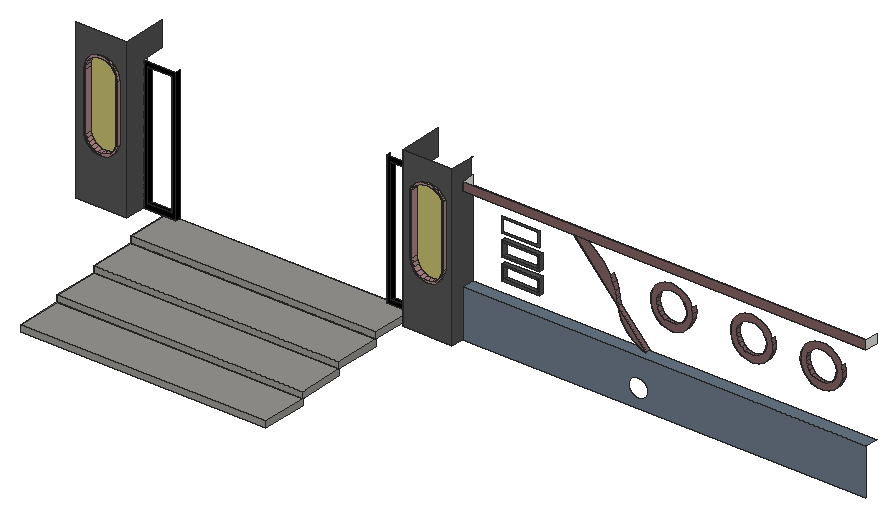
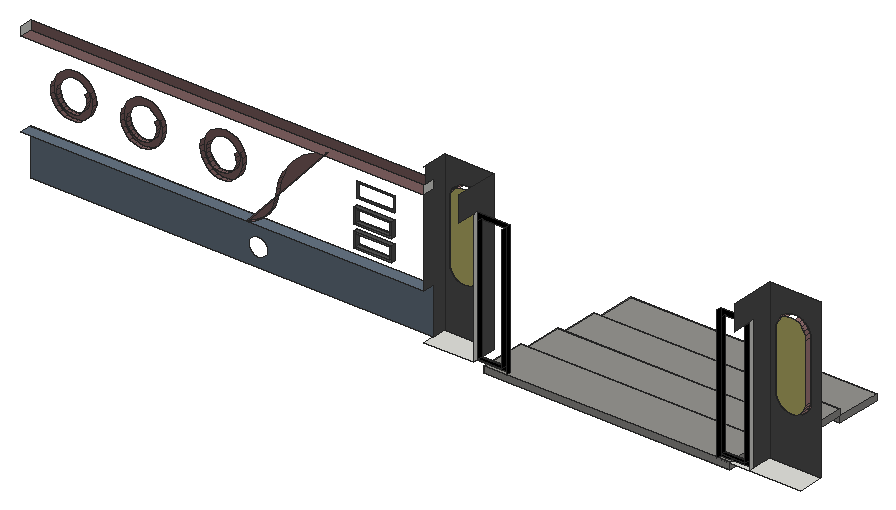
# SketchUp Ruby script. Lengths in inches.
U = 1.inch
M = Sketchup.active_model
def pt(a) = Geom::Point3d.new(a.map { |v| v * U })
def face(e, loops, mat)
  f = e.add_face(loops[0].map { |a| pt(a) })
  loops[1..].each { |l| e.add_face(l.map { |a| pt(a) }).erase! }
  f.material = f.back_material = mat if mat
  f
end
# faces: each face lists its corners as indices into pts; further lists are holes
def faces(e, pts, list, mat = nil) = list.each { |f| face(e, (f[0].is_a?(Array) ? f : [f]).map { |l| l.map { |i| pts[i] } }, mat) }
# xy, xz, yz: faces in a plane at the given z, y or x. An outline is a flat list of corners, or four numbers for a rectangle; further outlines are holes
def ring(l) = l.size == 4 ? [[l[0], l[1]], [l[2], l[1]], [l[2], l[3]], [l[0], l[3]]] : l.each_slice(2).to_a
def flat(e, list, mat, &to3) = list.each { |f| face(e, (f[0].is_a?(Array) ? f : [f]).map { |l| ring(l).map { |u, v| to3.(u, v) } }, mat) }
def xy(e, z, list, mat = nil) = flat(e, list, mat) { |x, y| [x, y, z] }
def xz(e, y, list, mat = nil) = flat(e, list, mat) { |x, z| [x, y, z] }
def yz(e, x, list, mat = nil) = flat(e, list, mat) { |y, z| [x, y, z] }
def lines(e, pts, list) = list.each { |a, b| e.add_line(pt(pts[a]), pt(pts[b])) }
# prism: a flat outline (further loops are holes) pulled along v
def prism(e, loops, v, mat = nil)
  f = face(e, loops, mat); d = Geom::Vector3d.new(v.map { |x| x * U })
  f.pushpull(f.normal.samedirection?(d) ? d.length : -d.length)
end
def box(e, o, s, mat = nil) = prism(e, [[o, [o[0] + s[0], o[1], o[2]], [o[0] + s[0], o[1] + s[1], o[2]], [o[0], o[1] + s[1], o[2]]]], [0, 0, s[2]], mat)
def at(x, y, z, deg = 0) = Geom::Transformation.translation(pt([x, y, z])) * Geom::Transformation.rotation(ORIGIN, Z_AXIS, deg.degrees)
def axes(o, x, y, z) = Geom::Transformation.new([*x, 0, *y, 0, *z, 0, *pt(o).to_a, 1])
def part(name) = M.definitions.add(name)
# library, detail: a bought-in or finely detailed component or shape, given as its bounding box
def library(name, o, s) = part(name).tap { |d| box(d.entities, o, s) }
def detail(e, o, s) = box(e.add_group.entities, o, s)
def put(e, d, t, mat = nil) = e.add_instance(d, t).tap { |i| i.material = mat if mat }
def group(e, t, mat = nil) = e.add_group.tap { |g| g.transformation = t; g.material = mat if mat }.entities
root = M.entities
M.materials.add("[0057_DarkKhaki]1").color = [189, 183, 107]
M.materials.add("[0111_SlateGray]").color = [103, 117, 132]
M.materials.add("[0119_RosyBrown]1").color = [124, 95, 95]
M.materials.add("[0119_RosyBrown]2").color = [170, 129, 129]
M.materials.add("[0135_DarkGray]").color = [81, 81, 81]
M.materials.add("[0137_Black]").color = [0, 0, 0]
M.materials.add("[Granite Light Gray]").color = [149, 148, 144]
xy(root,0,[[7,639.11,31.33,651.11],[162.58,639.11,186.0625,651.11],[31.33,649.11,46.92,651.11]])
xy(root,2.07,[[149.02,649.11,160.48,651.11]],"[0137_Black]")
xy(root,2.3,[[33.63,649.11,44.62,651.11]],"[0137_Black]")
xy(root,22.19,[[186.0625,645.11,377.9375,651.11]],"[0111_SlateGray]")
xy(root,28.6875,[[201.56,649.11,219.5,651.11]],"[0135_DarkGray]")
xy(root,29.54,[[202.42,649.11,218.64,651.11]],"[0135_DarkGray]")
xy(root,35.08,[[202.42,649.11,218.64,651.11]],"[0135_DarkGray]")
xy(root,35.9375,[[201.56,649.11,219.5,651.11]],"[0135_DarkGray]")
xy(root,38.875,[[201.56,649.11,219.5,651.11]],"[0135_DarkGray]")
xy(root,39.62,[[202.31,649.11,218.75,651.11]],"[0135_DarkGray]")
xy(root,45.375,[[202.31,649.11,218.75,651.11]],"[0135_DarkGray]")
xy(root,46.125,[[201.56,649.11,219.5,651.11]],"[0135_DarkGray]")
xy(root,63,[[186.0625,645.11,377.9375,651.11]],"[0119_RosyBrown]1")
xz(root,638.11,[[[19.87,22.97,21.71,23.18,23.47,23.8,25.04,24.79,26.34,26.11,27.32,27.6875,27.94,29.49,27.94,57.27,27.67,59.36,26.86,61.31,25.58,62.98,23.9,64.26,21.96,65.07,19.87,65.35,17.78,65.07,15.83,64.26,14.16,62.98,12.875,61.31,12.07,59.36,11.79,57.27,11.79,29.49,12.41,27.6875,13.39,26.11,14.7,24.79,16.27,23.8,18.02,23.18],[19.87,23.86,18.22,24.05,16.66,24.6,15.26,25.49,14.09,26.66,13.22,28.07,12.68,29.64,12.68,57.27,12.92,59.13,13.64,60.87,14.79,62.35,16.27,63.5,18.01,64.21,19.87,64.46,21.73,64.21,23.46,63.5,24.95,62.35,26.09,60.87,26.81,59.13,27.05,57.27,27.05,29.64,26.52,28.07,25.64,26.66,24.48,25.49,23.08,24.6,21.51,24.05]],[[174.87,23.28,176.93,23.55,178.86,24.35,180.51,25.62,181.78,27.27,182.58,29.19,182.85,31.26,182.85,60.6,181.89,62.1,180.79,63.28,179.49,64.24,178.04,64.95,176.48,65.39,174.87,65.54,173.26,65.39,171.7,64.95,170.25,64.24,168.95,63.28,167.84,62.1,166.88,60.6,166.88,31.26,167.16,29.19,167.95,27.27,169.22,25.62,170.875,24.35,172.8,23.55],[174.87,24.07,173.01,24.32,171.27,25.04,169.79,26.18,168.64,27.67,167.92,29.4,167.68,31.26,167.68,60.37,168.47,61.61,169.48,62.68,170.66,63.56,171.98,64.21,173.4,64.6,174.87,64.74,176.33,64.6,177.75,64.21,179.07,63.56,180.26,62.68,181.26,61.61,182.05,60.37,182.05,31.26,181.81,29.4,181.09,27.67,179.95,26.18,178.46,25.04,176.73,24.32]]],"[0119_RosyBrown]2")
xz(root,639.11,[[[7,0,31.33,75],[19.87,22.97,18.02,23.18,16.27,23.8,14.7,24.79,13.39,26.11,12.41,27.6875,11.79,29.49,11.79,57.27,12.07,59.36,12.875,61.31,14.16,62.98,15.83,64.26,17.78,65.07,19.87,65.35,21.96,65.07,23.9,64.26,25.58,62.98,26.86,61.31,27.67,59.36,27.94,57.27,27.94,29.49,27.32,27.6875,26.34,26.11,25.04,24.79,23.47,23.8,21.71,23.18]],[[162.58,0,186.0625,75],[174.87,23.28,172.8,23.55,170.875,24.35,169.22,25.62,167.95,27.27,167.16,29.19,166.88,31.26,166.88,60.6,167.84,62.1,168.95,63.28,170.25,64.24,171.7,64.95,173.26,65.39,174.87,65.54,176.48,65.39,178.04,64.95,179.49,64.24,180.79,63.28,181.89,62.1,182.85,60.6,182.85,31.26,182.58,29.19,181.78,27.27,180.51,25.62,178.86,24.35,176.93,23.55]]],"[0135_DarkGray]")
xz(root,641.11,[[19.87,23.86,21.51,24.05,23.08,24.6,24.48,25.49,25.64,26.66,26.52,28.07,27.05,29.64,27.05,57.27,26.81,59.13,26.09,60.87,24.95,62.35,23.46,63.5,21.73,64.21,19.87,64.46,18.01,64.21,16.27,63.5,14.79,62.35,13.64,60.87,12.92,59.13,12.68,57.27,12.68,29.64,13.22,28.07,14.09,26.66,15.26,25.49,16.66,24.6,18.22,24.05],[174.87,24.07,176.73,24.32,178.46,25.04,179.95,26.18,181.09,27.67,181.81,29.4,182.05,31.26,182.05,60.37,181.26,61.61,180.26,62.68,179.07,63.56,177.75,64.21,176.33,64.6,174.87,64.74,173.4,64.6,171.98,64.21,170.66,63.56,169.48,62.68,168.47,61.61,167.68,60.37,167.68,31.26,167.92,29.4,168.64,27.67,169.79,26.18,171.27,25.04,173.01,24.32]],"[0057_DarkKhaki]1")
xz(root,645.11,[[[186.0625,0,377.9375,22.19],[269.68,4.18,268.52,4.33,267.43,4.78,266.5,5.5,265.79,6.43,265.34,7.52,265.18,8.68,265.34,9.85,265.79,10.93,266.5,11.86,267.43,12.58,268.52,13.03,269.68,13.18,270.85,13.03,271.93,12.58,272.87,11.86,273.58,10.93,274.03,9.85,274.18,8.68,274.03,7.52,273.58,6.43,272.87,5.5,271.93,4.78,270.85,4.33]]],"[0111_SlateGray]")
xz(root,645.11,[[186.0625,63,377.9375,67.2]],"[0119_RosyBrown]1")
xz(root,649.11,[[270.01,22.19,270.11,22.28,256.72,37.33,256.61,37.24,256.97,35.5,257.5,33.8125,258.1875,32.18,259.02,30.61,260,29.14,261.12,27.76,262.36,26.49,263.71,25.35,265.17,24.34,266.71,23.47,268.33,22.75],[[282.96,35.68,285.56,36.18,287.93,37.34,289.93,39.07,291.41,41.26,292.27,43.76,292.46,46.4,291.95,48.99,290.8,51.37,289.0625,53.37,286.875,54.85,284.375,55.71,281.74,55.9,279.14,55.39,276.77,54.24,274.77,52.5,273.29,50.3125,272.43,47.8125,272.24,45.18,272.75,42.58,273.9,40.21,275.64,38.21,277.83,36.73,280.32,35.87],[282.78,38.68,280.92,38.81,279.17,39.41,277.625,40.46,276.41,41.86,275.59,43.53,275.24,45.36,275.37,47.21,275.98,48.97,277.02,50.51,278.42,51.73,280.09,52.55,281.92,52.9,283.77,52.77,285.53,52.16,287.07,51.12,288.29,49.72,289.11,48.04,289.46,46.22,289.33,44.36,288.72,42.6,287.68,41.0625,286.28,39.84,284.61,39.03]],[[320.9,35.68,323.49,36.18,325.87,37.34,327.87,39.07,329.35,41.26,330.21,43.76,330.39,46.4,329.89,48.99,328.73,51.37,327,53.37,324.8125,54.85,322.3125,55.71,319.68,55.9,317.08,55.39,314.7,54.24,312.71,52.5,311.23,50.3125,310.37,47.8125,310.18,45.18,310.68,42.58,311.84,40.21,313.57,38.21,315.76,36.73,318.26,35.87],[320.72,38.68,318.86,38.81,317.1,39.41,315.5625,40.46,314.34,41.86,313.53,43.53,313.18,45.36,313.31,47.21,313.91,48.97,314.95,50.51,316.36,51.73,318.03,52.55,319.86,52.9,321.71,52.77,323.47,52.16,325.01,51.12,326.23,49.72,327.05,48.04,327.4,46.22,327.27,44.36,326.66,42.6,325.62,41.0625,324.22,39.84,322.54,39.03]],[[354.15,35.68,356.74,36.18,359.12,37.34,361.12,39.07,362.6,41.26,363.46,43.76,363.64,46.4,363.14,48.99,361.98,51.37,360.25,53.37,358.0625,54.85,355.5625,55.71,352.93,55.9,350.33,55.39,347.95,54.24,345.96,52.5,344.48,50.3125,343.62,47.8125,343.43,45.18,343.93,42.58,345.09,40.21,346.82,38.21,349.01,36.73,351.51,35.87],[353.97,38.68,352.11,38.81,350.35,39.41,348.8125,40.46,347.59,41.86,346.78,43.53,346.43,45.36,346.56,47.21,347.16,48.97,348.2,50.51,349.61,51.73,351.28,52.55,353.11,52.9,354.96,52.77,356.72,52.16,358.26,51.12,359.48,49.72,360.3,48.04,360.65,46.22,360.52,44.36,359.91,42.6,358.87,41.0625,357.47,39.84,355.79,39.03]],[256.61,37.24,256.26,40.32,255.56,43.34,254.54,46.26,253.19,49.06,251.55,51.68,249.62,54.11,247.43,56.31,245.01,58.24,242.39,59.9,239.6,61.26,236.68,62.29,233.66,63]],"[0119_RosyBrown]1")
xz(root,649.11,[[[201.56,28.6875,219.5,35.9375],[202.42,29.54,218.64,35.08]],[[201.56,38.875,219.5,46.125],[202.31,39.62,218.75,45.375]],[[201.56,49.0625,219.5,56.3125],[202.32,49.82,218.74,55.55]]],"[0135_DarkGray]")
xz(root,649.11,[[[31.33,0,46.92,63],[33.63,2.3,44.62,60.7]],[[146.95,0,162.54,63],[149.02,2.07,160.48,60.93]]],"[0137_Black]")
yz(root,11.79,[[638.11,29.49,639.11,57.27]])
yz(root,12.68,[[638.11,29.64,641.11,57.27]],"[0119_RosyBrown]2")
yz(root,27.05,[[638.11,29.64,641.11,57.27]],"[0119_RosyBrown]2")
yz(root,27.94,[[638.11,29.49,639.11,57.27]],"[0119_RosyBrown]2")
yz(root,31.33,[[649.11,0,651.11,63]])
yz(root,31.33,[[639.11,0,649.11,0,649.11,63,660.11,63,660.11,75,639.11,75]],"[0135_DarkGray]")
yz(root,33.63,[[649.11,2.3,651.11,60.7]],"[0137_Black]")
yz(root,44.62,[[649.11,2.3,651.11,60.7]],"[0137_Black]")
yz(root,46.92,[[649.11,0,651.11,63]],"[0137_Black]")
yz(root,146.95,[[649.11,0,651.11,63]],"[0137_Black]")
yz(root,149.02,[[649.11,2.07,651.11,60.93]],"[0137_Black]")
yz(root,160.48,[[649.11,2.07,651.11,60.93]],"[0137_Black]")
yz(root,162.54,[[649.11,0,651.11,63]])
yz(root,162.58,[[639.11,0,639.11,75,660.11,75,660.11,63,651.11,63,651.11,0]],"[0135_DarkGray]")
yz(root,166.88,[[638.11,31.26,639.11,60.6]],"[0119_RosyBrown]2")
yz(root,167.68,[[638.11,31.26,641.11,60.37]],"[0119_RosyBrown]2")
yz(root,182.05,[[638.11,31.26,641.11,60.37]],"[0119_RosyBrown]2")
yz(root,182.85,[[638.11,31.26,639.11,60.6]],"[0119_RosyBrown]2")
yz(root,186.0625,[[645.11,63,651.11,67.2]])
yz(root,186.0625,[[639.11,0,645.11,0,645.11,22.19,651.11,22.19,651.11,63,645.11,63,645.11,67.2,650.11,67.2,650.11,74.96,651.11,74.96,651.11,75,639.11,75]],"[0135_DarkGray]")
yz(root,201.56,[[649.11,28.6875,651.11,35.9375],[649.11,38.875,651.11,46.125]],"[0135_DarkGray]")
yz(root,202.31,[[649.11,39.62,651.11,45.375]],"[0135_DarkGray]")
yz(root,202.42,[[649.11,29.54,651.11,35.08]],"[0135_DarkGray]")
yz(root,218.64,[[649.11,29.54,651.11,35.08]],"[0135_DarkGray]")
yz(root,218.75,[[649.11,39.62,651.11,45.375]],"[0135_DarkGray]")
yz(root,219.5,[[649.11,28.6875,651.11,35.9375],[649.11,38.875,651.11,46.125]],"[0135_DarkGray]")
yz(root,377.9375,[[645.11,63,651.11,67.2]])
p = [[268.33,651.11,22.75],[270.01,651.11,22.19],[270.01,649.11,22.19],[268.33,649.11,22.75],[270.11,651.11,22.28],[270.11,649.11,22.28],
  [256.72,651.11,37.33],[256.72,649.11,37.33],[266.71,651.11,23.47],[266.71,649.11,23.47],[18.02,639.11,23.18],[19.87,639.11,22.97],
  [19.87,638.11,22.97],[18.02,638.11,23.18],[21.71,639.11,23.18],[21.71,638.11,23.18],[16.27,639.11,23.8],[16.27,638.11,23.8],
  [23.47,639.11,23.8],[23.47,638.11,23.8],[172.8,639.11,23.55],[174.87,639.11,23.28],[174.87,638.11,23.28],[172.8,638.11,23.55],
  [176.93,639.11,23.55],[176.93,638.11,23.55],[170.875,639.11,24.35],[170.875,638.11,24.35],[178.86,639.11,24.35],[178.86,638.11,24.35],
  [265.17,651.11,24.34],[265.17,649.11,24.34],[14.7,639.11,24.79],[14.7,638.11,24.79],[25.04,639.11,24.79],[25.04,638.11,24.79],
  [18.22,641.11,24.05],[18.22,638.11,24.05],[19.87,638.11,23.86],[19.87,641.11,23.86],[21.51,638.11,24.05],[21.51,641.11,24.05],
  [16.66,641.11,24.6],[16.66,638.11,24.6],[23.08,638.11,24.6],[23.08,641.11,24.6],[173.01,641.11,24.32],[173.01,638.11,24.32],
  [174.87,638.11,24.07],[174.87,641.11,24.07],[176.73,638.11,24.32],[176.73,641.11,24.32],[169.22,639.11,25.62],[169.22,638.11,25.62],
  [171.27,641.11,25.04],[171.27,638.11,25.04],[178.46,638.11,25.04],[178.46,641.11,25.04],[180.51,639.11,25.62],[180.51,638.11,25.62],
  [263.71,651.11,25.35],[263.71,649.11,25.35],[15.26,641.11,25.49],[15.26,638.11,25.49],[24.48,638.11,25.49],[24.48,641.11,25.49],
  [13.39,639.11,26.11],[13.39,638.11,26.11],[26.34,639.11,26.11],[26.34,638.11,26.11],[169.79,641.11,26.18],[169.79,638.11,26.18],
  [179.95,638.11,26.18],[179.95,641.11,26.18],[262.36,651.11,26.49],[262.36,649.11,26.49],[14.09,641.11,26.66],[14.09,638.11,26.66],
  [25.64,638.11,26.66],[25.64,641.11,26.66],[167.95,639.11,27.27],[167.95,638.11,27.27],[181.78,639.11,27.27],[181.78,638.11,27.27],
  [12.41,639.11,27.6875],[12.41,638.11,27.6875],[27.32,639.11,27.6875],[27.32,638.11,27.6875],[168.64,641.11,27.67],[168.64,638.11,27.67],
  [181.09,638.11,27.67],[181.09,641.11,27.67],[261.12,651.11,27.76],[261.12,649.11,27.76],[13.22,641.11,28.07],[13.22,638.11,28.07],
  [26.52,638.11,28.07],[26.52,641.11,28.07],[167.16,639.11,29.19],[167.16,638.11,29.19],[182.58,639.11,29.19],[182.58,638.11,29.19],
  [11.79,639.11,29.49],[11.79,638.11,29.49],[27.94,639.11,29.49],[27.94,638.11,29.49],[167.92,641.11,29.4],[167.92,638.11,29.4],
  [181.81,638.11,29.4],[181.81,641.11,29.4],[260,651.11,29.14],[260,649.11,29.14],[12.68,641.11,29.64],[12.68,638.11,29.64],
  [27.05,638.11,29.64],[27.05,641.11,29.64],[259.02,651.11,30.61],[259.02,649.11,30.61],[166.88,639.11,31.26],[166.88,638.11,31.26],
  [182.85,639.11,31.26],[182.85,638.11,31.26],[167.68,641.11,31.26],[167.68,638.11,31.26],[182.05,638.11,31.26],[182.05,641.11,31.26],
  [258.1875,651.11,32.18],[258.1875,649.11,32.18],[257.5,651.11,33.8125],[257.5,649.11,33.8125],[256.97,651.11,35.5],[256.97,649.11,35.5],
  [256.61,651.11,37.24],[256.61,649.11,37.24],[280.32,651.11,35.87],[282.96,651.11,35.68],[282.96,649.11,35.68],[280.32,649.11,35.87],
  [285.56,651.11,36.18],[285.56,649.11,36.18],[318.26,651.11,35.87],[320.9,651.11,35.68],[320.9,649.11,35.68],[318.26,649.11,35.87],
  [323.49,651.11,36.18],[323.49,649.11,36.18],[351.51,651.11,35.87],[354.15,651.11,35.68],[354.15,649.11,35.68],[351.51,649.11,35.87],
  [356.74,651.11,36.18],[356.74,649.11,36.18],[277.83,651.11,36.73],[277.83,649.11,36.73],[315.76,651.11,36.73],[315.76,649.11,36.73],
  [349.01,651.11,36.73],[349.01,649.11,36.73],[287.93,651.11,37.34],[287.93,649.11,37.34],[325.87,651.11,37.34],[325.87,649.11,37.34],
  [359.12,651.11,37.34],[359.12,649.11,37.34],[275.64,651.11,38.21],[275.64,649.11,38.21],[313.57,651.11,38.21],[313.57,649.11,38.21],
  [346.82,651.11,38.21],[346.82,649.11,38.21],[233.66,651.11,63],[233.66,649.11,63],[256.26,651.11,40.32],[256.26,649.11,40.32],
  [289.93,651.11,39.07],[289.93,649.11,39.07],[327.87,651.11,39.07],[327.87,649.11,39.07],[361.12,651.11,39.07],[361.12,649.11,39.07],
  [273.9,651.11,40.21],[273.9,649.11,40.21],[311.84,651.11,40.21],[311.84,649.11,40.21],[345.09,651.11,40.21],[345.09,649.11,40.21],
  [282.78,651.11,38.68],[280.92,651.11,38.81],[280.92,649.11,38.81],[282.78,649.11,38.68],[284.61,651.11,39.03],[284.61,649.11,39.03],
  [320.72,651.11,38.68],[318.86,651.11,38.81],[318.86,649.11,38.81],[320.72,649.11,38.68],[322.54,651.11,39.03],[322.54,649.11,39.03],
  [353.97,651.11,38.68],[352.11,651.11,38.81],[352.11,649.11,38.81],[353.97,649.11,38.68],[355.79,651.11,39.03],[355.79,649.11,39.03],
  [279.17,651.11,39.41],[279.17,649.11,39.41],[317.1,651.11,39.41],[317.1,649.11,39.41],[350.35,651.11,39.41],[350.35,649.11,39.41],
  [286.28,651.11,39.84],[286.28,649.11,39.84],[324.22,651.11,39.84],[324.22,649.11,39.84],[357.47,651.11,39.84],[357.47,649.11,39.84],
  [291.41,651.11,41.26],[291.41,649.11,41.26],[329.35,651.11,41.26],[329.35,649.11,41.26],[362.6,651.11,41.26],[362.6,649.11,41.26],
  [277.625,651.11,40.46],[277.625,649.11,40.46],[315.5625,651.11,40.46],[315.5625,649.11,40.46],[348.8125,651.11,40.46],[348.8125,649.11,40.46],
  [287.68,651.11,41.0625],[287.68,649.11,41.0625],[325.62,651.11,41.0625],[325.62,649.11,41.0625],[358.87,651.11,41.0625],[358.87,649.11,41.0625],
  [272.75,651.11,42.58],[272.75,649.11,42.58],[310.68,651.11,42.58],[310.68,649.11,42.58],[343.93,651.11,42.58],[343.93,649.11,42.58],
  [255.56,651.11,43.34],[255.56,649.11,43.34],[276.41,651.11,41.86],[276.41,649.11,41.86],[314.34,651.11,41.86],[314.34,649.11,41.86],
  [347.59,651.11,41.86],[347.59,649.11,41.86],[288.72,651.11,42.6],[288.72,649.11,42.6],[326.66,651.11,42.6],[326.66,649.11,42.6],
  [359.91,651.11,42.6],[359.91,649.11,42.6],[292.27,651.11,43.76],[292.27,649.11,43.76],[330.21,651.11,43.76],[330.21,649.11,43.76],
  [363.46,651.11,43.76],[363.46,649.11,43.76],[275.59,651.11,43.53],[275.59,649.11,43.53],[313.53,651.11,43.53],[313.53,649.11,43.53],
  [346.78,651.11,43.53],[346.78,649.11,43.53],[272.24,651.11,45.18],[272.24,649.11,45.18],[289.33,651.11,44.36],[289.33,649.11,44.36],
  [310.18,651.11,45.18],[310.18,649.11,45.18],[327.27,651.11,44.36],[327.27,649.11,44.36],[343.43,651.11,45.18],[343.43,649.11,45.18],
  [360.52,651.11,44.36],[360.52,649.11,44.36],[254.54,651.11,46.26],[254.54,649.11,46.26],[275.24,651.11,45.36],[275.24,649.11,45.36],
  [313.18,651.11,45.36],[313.18,649.11,45.36],[346.43,651.11,45.36],[346.43,649.11,45.36],[292.46,651.11,46.4],[292.46,649.11,46.4],
  [330.39,651.11,46.4],[330.39,649.11,46.4],[363.64,651.11,46.4],[363.64,649.11,46.4],[289.46,651.11,46.22],[289.46,649.11,46.22],
  [327.4,651.11,46.22],[327.4,649.11,46.22],[360.65,651.11,46.22],[360.65,649.11,46.22],[272.43,651.11,47.8125],[272.43,649.11,47.8125],
  [310.37,651.11,47.8125],[310.37,649.11,47.8125],[343.62,651.11,47.8125],[343.62,649.11,47.8125],[275.37,651.11,47.21],[275.37,649.11,47.21],
  [313.31,651.11,47.21],[313.31,649.11,47.21],[346.56,651.11,47.21],[346.56,649.11,47.21],[289.11,651.11,48.04],[289.11,649.11,48.04],
  [327.05,651.11,48.04],[327.05,649.11,48.04],[360.3,651.11,48.04],[360.3,649.11,48.04],[253.19,651.11,49.06],[253.19,649.11,49.06],
  [291.95,651.11,48.99],[291.95,649.11,48.99],[329.89,651.11,48.99],[329.89,649.11,48.99],[363.14,651.11,48.99],[363.14,649.11,48.99],
  [275.98,651.11,48.97],[275.98,649.11,48.97],[313.91,651.11,48.97],[313.91,649.11,48.97],[347.16,651.11,48.97],[347.16,649.11,48.97],
  [273.29,651.11,50.3125],[273.29,649.11,50.3125],[311.23,651.11,50.3125],[311.23,649.11,50.3125],[344.48,651.11,50.3125],[344.48,649.11,50.3125],
  [288.29,651.11,49.72],[288.29,649.11,49.72],[12.07,639.11,59.36],[11.79,639.11,57.27],[11.79,638.11,57.27],[12.07,638.11,59.36],
  [12.92,641.11,59.13],[12.92,638.11,59.13],[12.68,638.11,57.27],[12.68,641.11,57.27],[27.05,641.11,57.27],[27.05,638.11,57.27],
  [26.81,638.11,59.13],[26.81,641.11,59.13],[27.94,639.11,57.27],[27.67,639.11,59.36],[27.67,638.11,59.36],[27.94,638.11,57.27],
  [13.64,641.11,60.87],[13.64,638.11,60.87],[26.09,638.11,60.87],[26.09,641.11,60.87],[12.875,639.11,61.31],[12.875,638.11,61.31],
  [26.86,639.11,61.31],[26.86,638.11,61.31],[168.47,641.11,61.61],[168.47,638.11,61.61],[167.68,638.11,60.37],[167.68,641.11,60.37],
  [182.05,641.11,60.37],[182.05,638.11,60.37],[181.26,638.11,61.61],[181.26,641.11,61.61],[167.84,639.11,62.1],[166.88,639.11,60.6],
  [166.88,638.11,60.6],[167.84,638.11,62.1],[182.85,639.11,60.6],[181.89,639.11,62.1],[181.89,638.11,62.1],[182.85,638.11,60.6],
  [14.79,641.11,62.35],[14.79,638.11,62.35],[24.95,638.11,62.35],[24.95,641.11,62.35],[14.16,639.11,62.98],[14.16,638.11,62.98],
  [25.58,639.11,62.98],[25.58,638.11,62.98],[169.48,641.11,62.68],[169.48,638.11,62.68],[180.26,638.11,62.68],[180.26,641.11,62.68],
  [168.95,639.11,63.28],[168.95,638.11,63.28],[180.79,639.11,63.28],[180.79,638.11,63.28],[16.27,641.11,63.5],[16.27,638.11,63.5],
  [23.46,638.11,63.5],[23.46,641.11,63.5],[170.66,641.11,63.56],[170.66,638.11,63.56],[179.07,638.11,63.56],[179.07,641.11,63.56],
  [15.83,639.11,64.26],[15.83,638.11,64.26],[23.9,639.11,64.26],[23.9,638.11,64.26],[170.25,639.11,64.24],[170.25,638.11,64.24],
  [179.49,639.11,64.24],[179.49,638.11,64.24],[18.01,641.11,64.21],[18.01,638.11,64.21],[21.73,638.11,64.21],[21.73,641.11,64.21],
  [171.98,641.11,64.21],[171.98,638.11,64.21],[177.75,638.11,64.21],[177.75,641.11,64.21]]
faces(root,p,[[0,1,2,3],[4,6,7,5],[8,0,3,9],[30,8,9,31],[60,30,31,61],[74,60,61,75],[92,74,75,93],[110,92,93,111],
  [116,110,111,117],[126,116,117,127],[128,126,127,129],[130,128,129,131],[132,130,131,133],[134,135,136,137],[135,138,139,136],[140,141,142,143],
  [141,144,145,142],[146,147,148,149],[147,150,151,148],[152,134,137,153],[154,140,143,155],[156,146,149,157],[138,158,159,139],[144,160,161,145],
  [150,162,163,151],[164,152,153,165],[166,154,155,167],[168,156,157,169],[170,132,133,171],[132,172,173,133],[158,174,175,159],[160,176,177,161],
  [162,178,179,163],[180,164,165,181],[182,166,167,183],[184,168,169,185],[186,187,188,189],[190,186,189,191],[192,193,194,195],[196,192,195,197],
  [198,199,200,201],[202,198,201,203],[187,204,205,188],[193,206,207,194],[199,208,209,200],[210,190,191,211],[212,196,197,213],[214,202,203,215],
  [174,216,217,175],[176,218,219,177],[178,220,221,179],[204,222,223,205],[206,224,225,207],[208,226,227,209],[228,210,211,229],[230,212,213,231],
  [232,214,215,233],[234,180,181,235],[236,182,183,237],[238,184,185,239],[172,240,241,173],[222,242,243,223],[224,244,245,225],[226,246,247,227],
  [248,228,229,249],[250,230,231,251],[252,232,233,253],[216,254,255,217],[218,256,257,219],[220,258,259,221],[242,260,261,243],[244,262,263,245],
  [246,264,265,247],[266,234,235,267],[268,248,249,269],[270,236,237,271],[272,250,251,273],[274,238,239,275],[276,252,253,277],[240,278,279,241],
  [260,280,281,261],[262,282,283,263],[264,284,285,265],[254,286,287,255],[256,288,289,257],[258,290,291,259],[292,268,269,293],[294,272,273,295],
  [296,276,277,297],[298,266,267,299],[300,270,271,301],[302,274,275,303],[280,304,305,281],[282,306,307,283],[284,308,309,285],[310,292,293,311],
  [312,294,295,313],[314,296,297,315],[278,316,317,279],[286,318,319,287],[288,320,321,289],[290,322,323,291],[304,324,325,305],[306,326,327,307],
  [308,328,329,309],[330,298,299,331],[332,300,301,333],[334,302,303,335],[336,310,311,337]],"[0119_RosyBrown]1")
faces(root,p,[[2,1,4,5],[132,133,7,6]])
faces(root,p,[[10,11,12,13],[11,14,15,12],[16,10,13,17],[14,18,19,15],[20,21,22,23],[21,24,25,22],[26,20,23,27],[24,28,29,25],
  [32,16,17,33],[18,34,35,19],[36,37,38,39],[39,38,40,41],[42,43,37,36],[41,40,44,45],[46,47,48,49],[49,48,50,51],
  [52,26,27,53],[54,55,47,46],[51,50,56,57],[28,58,59,29],[62,63,43,42],[45,44,64,65],[66,32,33,67],[34,68,69,35],
  [70,71,55,54],[57,56,72,73],[76,77,63,62],[65,64,78,79],[80,52,53,81],[58,82,83,59],[84,66,67,85],[68,86,87,69],
  [88,89,71,70],[73,72,90,91],[94,95,77,76],[79,78,96,97],[98,80,81,99],[82,100,101,83],[102,84,85,103],[86,104,105,87],
  [106,107,89,88],[91,90,108,109],[112,113,95,94],[97,96,114,115],[118,98,99,119],[100,120,121,101],[122,123,107,106],[109,108,124,125],
  [338,339,340,341],[342,343,344,345],[346,347,348,349],[350,351,352,353],[354,355,343,342],[349,348,356,357],[358,338,341,359],[351,360,361,352],
  [362,363,364,365],[366,367,368,369],[370,371,372,373],[374,375,376,377],[378,379,355,354],[357,356,380,381],[382,358,359,383],[360,384,385,361],
  [386,387,363,362],[369,368,388,389],[390,370,373,391],[375,392,393,376],[394,395,379,378],[381,380,396,397],[398,399,387,386],[389,388,400,401],
  [402,382,383,403],[384,404,405,385],[406,390,391,407],[392,408,409,393],[410,411,395,394],[397,396,412,413],[414,415,399,398],[401,400,416,417]],"[0119_RosyBrown]2")
g1 = group(root,at(41.06,563.86,-12),"[Granite Light Gray]")
xy(g1,0,[[0,0,116.625,21.8125]])
xy(g1,3,[[0,0,116.625,21.8125],[0,21.8125,116.625,43.625]])
xy(g1,6,[[0,21.8125,116.625,43.625],[0,43.625,116.625,65.4375]])
xy(g1,9,[[0,43.625,116.625,65.4375],[0,65.4375,116.625,87.25]])
xy(g1,12,[[0,65.4375,116.625,87.25]])
xz(g1,0,[[0,0,116.625,3]])
xz(g1,21.8125,[[0,0,116.625,3],[0,3,116.625,6]])
xz(g1,43.625,[[0,3,116.625,6],[0,6,116.625,9]])
xz(g1,65.4375,[[0,6,116.625,9],[0,9,116.625,12]])
xz(g1,87.25,[[0,9,116.625,12]])
yz(g1,0,[[0,0,21.8125,3],[21.8125,3,43.625,6],[43.625,6,65.4375,9],[65.4375,9,87.25,12]])
yz(g1,116.625,[[0,0,21.8125,3],[21.8125,3,43.625,6],[43.625,6,65.4375,9],[65.4375,9,87.25,12]])
